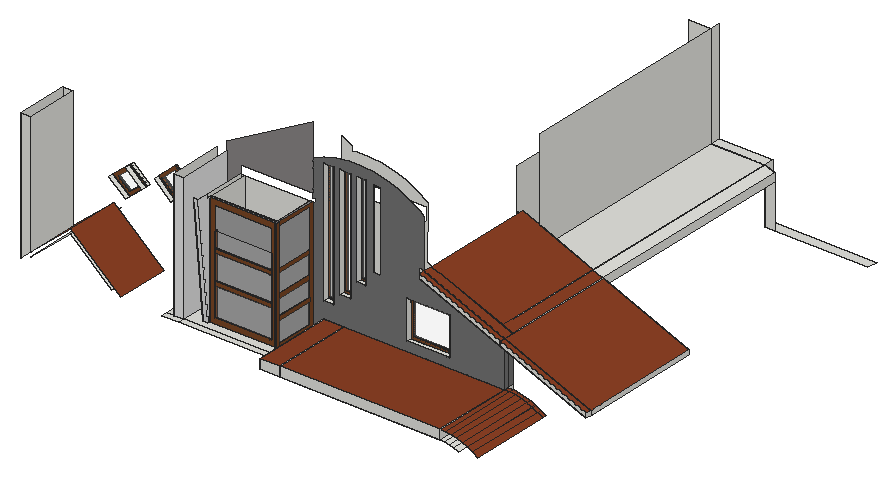
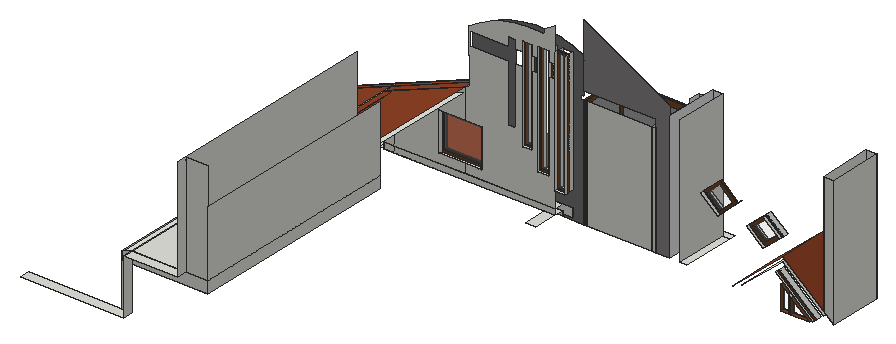
# SketchUp Ruby script. Lengths in inches.
U = 1.inch
M = Sketchup.active_model
def pt(a) = Geom::Point3d.new(a.map { |v| v * U })
def face(e, loops, mat)
  f = e.add_face(loops[0].map { |a| pt(a) })
  loops[1..].each { |l| e.add_face(l.map { |a| pt(a) }).erase! }
  f.material = f.back_material = mat if mat
  f
end
# faces: each face lists its corners as indices into pts; further lists are holes
def faces(e, pts, list, mat = nil) = list.each { |f| face(e, (f[0].is_a?(Array) ? f : [f]).map { |l| l.map { |i| pts[i] } }, mat) }
# xy, xz, yz: faces in a plane at the given z, y or x. An outline is a flat list of corners, or four numbers for a rectangle; further outlines are holes
def ring(l) = l.size == 4 ? [[l[0], l[1]], [l[2], l[1]], [l[2], l[3]], [l[0], l[3]]] : l.each_slice(2).to_a
def flat(e, list, mat, &to3) = list.each { |f| face(e, (f[0].is_a?(Array) ? f : [f]).map { |l| ring(l).map { |u, v| to3.(u, v) } }, mat) }
def xy(e, z, list, mat = nil) = flat(e, list, mat) { |x, y| [x, y, z] }
def xz(e, y, list, mat = nil) = flat(e, list, mat) { |x, z| [x, y, z] }
def yz(e, x, list, mat = nil) = flat(e, list, mat) { |y, z| [x, y, z] }
def lines(e, pts, list) = list.each { |a, b| e.add_line(pt(pts[a]), pt(pts[b])) }
# prism: a flat outline (further loops are holes) pulled along v
def prism(e, loops, v, mat = nil)
  f = face(e, loops, mat); d = Geom::Vector3d.new(v.map { |x| x * U })
  f.pushpull(f.normal.samedirection?(d) ? d.length : -d.length)
end
def box(e, o, s, mat = nil) = prism(e, [[o, [o[0] + s[0], o[1], o[2]], [o[0] + s[0], o[1] + s[1], o[2]], [o[0], o[1] + s[1], o[2]]]], [0, 0, s[2]], mat)
def at(x, y, z, deg = 0) = Geom::Transformation.translation(pt([x, y, z])) * Geom::Transformation.rotation(ORIGIN, Z_AXIS, deg.degrees)
def axes(o, x, y, z) = Geom::Transformation.new([*x, 0, *y, 0, *z, 0, *pt(o).to_a, 1])
def part(name) = M.definitions.add(name)
# library, detail: a bought-in or finely detailed component or shape, given as its bounding box
def library(name, o, s) = part(name).tap { |d| box(d.entities, o, s) }
def detail(e, o, s) = box(e.add_group.entities, o, s)
def put(e, d, t, mat = nil) = e.add_instance(d, t).tap { |i| i.material = mat if mat }
def group(e, t, mat = nil) = e.add_group.tap { |g| g.transformation = t; g.material = mat if mat }.entities
root = M.entities
M.materials.add("Glass Thin Clear 001").color = [243, 240, 240]
M.materials["Glass Thin Clear 001"].alpha = 0.1
M.materials.add("[Blinds Vertical Stripe Gray]").color = [160, 160, 160]
M.materials.add("[Brick Tumbled]").color = [135, 132, 132]
M.materials.add("[Color M01]").color = [226, 226, 226]
M.materials.add("[Color M05]").color = [114, 114, 114]
M.materials.add("[Roofing Tile Spanish]").color = [138, 64, 36]
M.materials.add("[Wood Veneer 01]").color = [120, 70, 37]
xy(root,124.49,[[41.61,170.5625,44.06,171.0625],[41.61,171.0625,44.06,173.875]])
xy(root,124.49,[[25.1,170.5625,41.61,171.0625],[44.06,170.5625,50.73,171.0625],[25.1,171.0625,41.61,173.875],[44.06,171.0625,50.73,173.875]],"[Wood Veneer 01]")
xy(root,126,[[141.15,112.5625,156.96,118.0625],[156.96,112.5625,252.96,118.0625],[141.15,118.0625,147.96,166.0625],[156.96,118.0625,252.96,118.0625,252.96,166.0625,233.59,166.0625,233.59,126.375,172.96,126.375,172.96,124.07,168.96,124.07,168.96,166.0625,156.96,166.0625],[252.96,118.0625,261.96,166.0625],
  [168.96,124.07,172.96,126.375],[168.96,126.375,172.96,166.0625],[172.96,126.375,231.27,128.3125],[231.84,126.375,233.59,128.3125],[172.96,128.3125,231.27,128.5625],
  [231.27,128.3125,231.84,128.5625],[231.84,128.3125,233.59,128.5625],[172.96,128.5625,231.27,128.9375],[172.96,128.9375,231.27,166.0625],[231.34,128.9375,231.84,166.0625]])
xy(root,126,[[231.27,126.375,231.84,128.3125],[231.27,128.5625,231.34,128.9375],[231.34,128.5625,231.84,128.9375],[231.84,128.5625,233.59,128.9375],[231.27,128.9375,231.34,166.0625],
  [231.84,128.9375,233.59,166.0625]],"[Wood Veneer 01]")
xy(root,127.6,[[244.09,93.6875,252.96,166.0625],[252.96,93.6875,261.96,118.0625],[261.96,93.6875,405.96,118.0625],[261.96,118.0625,405.96,166.0625]])
xy(root,128.55,[[231.27,128.93,233.15,163.51],[233.15,128.93,233.59,163.51]],"[Wood Veneer 01]")
xy(root,130.625,[[252.96,118.0625,261.96,166.0625],[261.96,118.0625,405.96,166.0625],[252.96,166.0625,261.96,175.0625],[261.96,166.0625,405.96,175.0625],[252.96,175.0625,261.96,196.0625],
  [396.96,469.0625,489.96,478.0625]])
xy(root,130.81,[[177.78,126.375,228.77,127],[177.78,127,228.77,128.9375]],"[Wood Veneer 01]")
xy(root,135.875,[[252.96,166.0625,333.96,175.0625],[333.96,166.0625,405.96,175.0625]])
xy(root,135.875,[[244.09,93.6875,261.96,166.0625],[261.96,93.6875,405.96,166.0625]],"[Roofing Tile Spanish]")
xy(root,144.3,[[318.48,166.0625,356.67,170.5625],[318.48,172.3125,356.67,175.0625]])
xy(root,144.3,[[318.48,170.5625,356.67,170.875],[318.48,170.875,356.67,171.8125],[318.48,171.8125,356.67,172.3125]],"[Wood Veneer 01]")
xy(root,146.54,[[320.73,170.5625,354.42,170.875],[320.73,170.875,354.42,172.3125]],"[Wood Veneer 01]")
xy(root,146.8,[[231.27,128.93,233.15,163.51],[233.15,128.93,233.59,163.51]],"[Wood Veneer 01]")
xy(root,150.38,[[231.27,128.93,233.15,163.51],[233.15,128.93,233.59,163.51]],"[Wood Veneer 01]")
xy(root,150.4,[[243.5625,166.0625,252.8125,170.5625],[243.5625,172.5,252.8125,175.0625]])
xy(root,150.4,[[243.5625,170.5625,252.8125,172.125],[243.5625,172.125,252.8125,172.5]],"[Wood Veneer 01]")
xy(root,151.26,[[244.43,170.5625,251.95,170.8125],[244.43,170.8125,251.95,172.5]],"[Wood Veneer 01]")
xy(root,156.93,[[177.78,126.375,228.77,127],[177.78,127,228.77,128.9375]],"[Wood Veneer 01]")
xy(root,160.3125,[[177.78,126.375,228.77,127],[177.78,127,228.77,128.9375]],"[Wood Veneer 01]")
xy(root,160.43,[[258.23,166.0625,268.1,170.5625],[258.23,170.5625,268.1,172.4375],[258.23,172.4375,268.1,172.5],[258.23,172.5,268.1,175.0625]])
xy(root,161.64,[[259.4375,170.5625,266.9,171.125],[259.4375,171.125,266.9,172.5]],"[Wood Veneer 01]")
xy(root,164.87,[[231.27,128.93,233.15,163.51],[233.15,128.93,233.59,163.51]],"[Wood Veneer 01]")
xy(root,168.44,[[231.27,128.93,233.15,163.51],[233.15,128.93,233.59,163.51]],"[Wood Veneer 01]")
xy(root,170.02,[[328.85,276.6875,396.96,469.0625],[396.96,276.6875,405.96,469.0625]])
xy(root,175.79,[[273.05,166.0625,281.55,170.5625],[273.05,170.5625,281.55,172.4375],[273.05,172.4375,281.55,172.5],[273.05,172.5,281.55,175.0625]])
xy(root,176.74,[[320.73,170.5625,354.42,170.875],[320.73,170.875,354.42,172.3125]],"[Wood Veneer 01]")
xy(root,176.78,[[274.03,170.5625,280.57,171.125],[274.03,171.125,280.57,172.5]],"[Wood Veneer 01]")
xy(root,177,[[396.96,175.0625,405.96,187.0625],[396.96,187.0625,405.96,276.6875]])
xy(root,178.98,[[318.48,166.0625,356.67,170.5625],[318.48,172.3125,356.67,175.0625]])
xy(root,178.98,[[318.48,170.5625,356.67,170.875],[318.48,170.875,356.67,171.8125],[318.48,171.8125,356.67,172.3125]],"[Wood Veneer 01]")
xy(root,180.58,[[328.85,276.6875,348.92,469.0625],[348.92,276.6875,396.96,469.0625],[348.92,469.0625,396.96,478.0625]])
xy(root,183.04,[[177.78,126.375,228.77,127],[177.78,127,228.77,128.9375]],"[Wood Veneer 01]")
xy(root,185.43,[[231.27,128.93,233.15,163.51],[233.15,128.93,233.59,163.51]],"[Wood Veneer 01]")
xy(root,186.43,[[177.78,126.375,228.77,127],[177.78,127,228.77,128.9375]],"[Wood Veneer 01]")
xz(root,93.6875,[[244.09,127.6,261.96,135.875],[261.96,127.6,405.96,135.875]])
xz(root,118.0625,[[9.96,124,18.96,131.72,18.96,240,9.96,240],[252.96,126,261.96,127.6],[252.96,127.6,261.96,130.625],[261.96,127.6,405.96,130.625]])
xz(root,118.0625,[[147.96,126,156.96,240]],"[Color M01]")
xz(root,126.375,[[168.96,126,172.96,226.125]])
xz(root,126.375,[[[172.96,126,231.27,226.125],[177.78,130.81,228.77,221.31]],[231.27,126,231.84,226.125],[231.84,126,233.59,226.125],[177.78,156.93,228.77,160.3125],[177.78,183.04,228.77,186.43]],"[Wood Veneer 01]")
xz(root,127,[[177.78,130.81,228.77,156.93],[177.78,160.3125,228.77,183.04],[177.78,186.43,228.77,200.48]],"Glass Thin Clear 001")
xz(root,128.3125,[[172.96,126,233.59,226.125]],"[Blinds Vertical Stripe Gray]")
xz(root,128.93,[[231.27,146.8,233.59,150.38],[231.27,164.87,233.59,168.44],[231.27,185.43,233.59,189.01]])
xz(root,128.93,[[231.27,128.55,233.15,146.8],[233.15,128.55,233.59,146.8],[231.27,150.38,233.15,164.87],[233.15,150.38,233.59,164.87],[231.27,168.44,233.15,185.43],
  [233.15,168.44,233.59,185.43]],"[Wood Veneer 01]")
xz(root,128.9375,[[[172.96,126,233.59,226.125],[177.78,130.81,228.77,221.31]],[177.78,156.93,228.77,160.3125],[177.78,183.04,228.77,186.43]],"[Wood Veneer 01]")
xz(root,161.1875,[[483.0625,142.27,483.0625,146.27,405.96,177,405.96,173],[405.96,173,405.96,177,333.96,205.6875,333.96,201.6875]])
xz(root,163.51,[[231.27,146.8,233.59,150.38],[231.27,164.87,233.59,168.44],[231.27,185.43,233.59,189.01]])
xz(root,163.51,[[231.27,128.55,233.15,146.8],[233.15,128.55,233.59,146.8],[231.27,150.38,233.15,164.87],[233.15,150.38,233.59,164.87],[231.27,168.44,233.15,185.43],
  [233.15,168.44,233.59,185.43]],"[Wood Veneer 01]")
xz(root,166.0625,[[9.96,124,9.96,240,18.96,240,18.96,131.72],[168.96,126,172.96,226.125],[172.96,126,231.27,226.125],[231.34,126,231.84,226.125],[252.96,126,261.96,130.625],
  [244.09,127.6,244.09,135.875,261.96,135.875,261.96,130.625,252.96,130.625,252.96,127.6],[261.96,127.6,405.96,130.625],[261.96,130.625,405.96,135.875],[483.0625,142.27,405.96,173,405.96,177,483.0625,146.27],[405.96,173,333.96,201.6875,333.96,205.6875,405.96,177]])
xz(root,166.0625,[[156.96,126,168.96,126,168.96,233.5,233.59,233.5,233.59,290.5,156.96,248]],"[Brick Tumbled]")
xz(root,166.0625,[[[233.59,126,252.96,126,252.96,127.6,244.09,127.6,244.09,135.875,405.96,135.875,405.96,173,333.96,201.6875,328.85,203.72,328.85,207.72,333.96,205.6875,333.96,249.1,329.8,252.53,320.33,258.625,310.2,263.55,299.57,267.25,288.57,269.67,277.36,270.78,266.11,270.55,261.96,269.97,254.95,268.99,252.96,268.47,244.0625,266.13,233.59,262,233.59,229.5625,236.34,229.5625,236.34,226.125,233.59,226.125],[318.48,144.3,356.67,178.98],[243.5625,150.4,252.8125,261.4],[258.23,160.43,268.1,261.18],[273.05,175.79,281.55,260.67],[288.03,188.71,295.34,259.58]]],"[Color M05]")
xz(root,166.0625,[[231.27,126,231.34,226.125],[231.84,126,233.59,226.125]],"[Wood Veneer 01]")
xz(root,170.5625,[[41.61,124.49,44.06,124.49,44.06,140.36,41.61,138.3],[[318.48,144.3,356.67,178.98],[320.73,146.54,354.42,176.74]],[[243.5625,150.4,252.8125,261.4],[244.43,151.26,251.95,260.53]],[[258.23,160.43,268.1,261.18],[259.4375,161.64,266.9,259.97]],[[66.04,170.09,80.79,182.43,66.04,194.78,51.29,182.43],[66.04,173.375,55.21,182.43,66.04,191.49,76.86,182.43]],
  [[273.05,175.79,281.55,260.67],[274.03,176.78,280.57,259.6875]],[[106.65,181.57,121.43,195.01,106.65,208.45,91.87,195.01],[106.65,184.29,94.86,195.01,106.65,205.73,118.44,195.01]]],"[Wood Veneer 01]")
xz(root,170.8125,[[244.43,151.26,251.95,260.53]],"Glass Thin Clear 001")
xz(root,170.875,[[[318.48,144.3,356.67,178.98],[320.73,146.54,354.42,176.74]]])
xz(root,170.875,[[320.73,146.54,354.42,176.74],[66.04,173.375,76.86,182.43,66.04,191.49,55.21,182.43],[106.65,184.29,118.44,195.01,106.65,205.73,94.86,195.01]],"Glass Thin Clear 001")
xz(root,171.0625,[[41.61,124.49,41.61,138.3,44.06,140.36,44.06,124.49]])
xz(root,171.0625,[[25.1,124.49,41.61,124.49,41.61,138.3],[44.06,124.49,50.73,124.49,50.73,145.9375,44.06,140.36]],"Glass Thin Clear 001")
xz(root,171.125,[[259.4375,161.64,266.9,259.97],[274.03,176.78,280.57,259.6875]],"Glass Thin Clear 001")
xz(root,171.8125,[[318.48,144.3,356.67,178.98]],"Glass Thin Clear 001")
xz(root,171.875,[[66.04,170.09,51.29,182.43,66.04,194.78,80.79,182.43],[106.65,181.57,91.87,195.01,106.65,208.45,121.43,195.01]],"Glass Thin Clear 001")
xz(root,172.125,[[243.5625,150.4,252.8125,261.4]],"Glass Thin Clear 001")
xz(root,172.3125,[[[318.48,144.3,356.67,178.98],[320.73,146.54,354.42,176.74]]],"[Wood Veneer 01]")
xz(root,172.4375,[[258.23,160.43,268.1,261.18],[273.05,175.79,281.55,260.67]],"Glass Thin Clear 001")
xz(root,172.4375,[[[66.04,170.09,51.29,182.43,66.04,194.78,80.79,182.43],[66.04,173.375,76.86,182.43,66.04,191.49,55.21,182.43]],[[106.65,181.57,91.87,195.01,106.65,208.45,121.43,195.01],[106.65,184.29,118.44,195.01,106.65,205.73,94.86,195.01]]],"[Wood Veneer 01]")
xz(root,172.5,[[[243.5625,150.4,252.8125,261.4],[244.43,151.26,251.95,260.53]],[[258.23,160.43,268.1,261.18],[259.4375,161.64,266.9,259.97]],[[273.05,175.79,281.55,260.67],[274.03,176.78,280.57,259.6875]]],"[Wood Veneer 01]")
xz(root,173.875,[[41.61,124.49,41.61,138.3,44.06,140.36,44.06,124.49]],"[Wood Veneer 01]")
xz(root,175.0625,[[252.96,130.625,396.96,135.875],[396.96,130.625,405.96,135.875],[252.96,135.875,252.96,240,258.23,240,258.23,160.43,268.1,160.43,268.1,240,273.05,240,273.05,175.79,281.55,175.79,281.55,240,288.03,240,288.03,188.71,295.34,188.71,295.34,240,328.85,240,328.85,252,295.34,252,295.34,259.58,288.03,259.58,288.03,252,281.55,252,281.55,260.67,273.05,260.67,273.05,252,268.1,252,268.1,261.18,258.23,261.18,258.23,252,252.96,252,252.96,282.53,261.96,276.98,261.96,272.98,266.11,273.55,277.36,273.78,288.57,272.68,299.57,270.26,310.2,266.5625,320.33,261.63,329.8,255.54,328.85,207.72,333.96,205.6875,333.96,178.98,318.48,178.98,318.48,144.3,333.96,144.3,333.96,135.875],[333.96,135.875,333.96,144.3,356.67,144.3,356.67,178.98,333.96,178.98,333.96,205.6875,396.96,180.58,396.96,135.875],[396.96,135.875,405.96,177],
  [396.96,177,405.96,177,396.96,180.58]])
xz(root,276.6875,[[483.0625,142.27,405.96,173,405.96,177,483.0625,146.27],[328.85,170.02,396.96,176.58],[396.96,170.02,405.96,170.02,405.96,173,396.96,176.58],[405.96,173,396.96,176.58,396.96,177,405.96,177],[328.85,176.58,396.96,176.58,395.92,177,328.85,177],
  [396.96,176.58,395.92,177,396.96,177],[328.85,177,395.92,177,386.92,180.58,328.85,180.58],[395.92,177,386.92,180.58,396.96,180.58,396.96,177],[396.96,177,405.96,177,396.96,180.58],[328.85,180.58,348.92,180.58,348.92,195.73,333.96,201.6875,328.85,203.72],
  [386.92,180.58,348.92,195.73,348.92,199.73,396.96,180.58]])
xz(root,469.0625,[[396.96,130.625,405.96,170.02],[328.85,170.02,396.96,180.58],[396.96,170.02,396.96,180.58,405.96,177,405.96,170.02],[328.85,180.58,348.92,272.68]])
yz(root,9.96,[[118.0625,124,166.0625,240]])
yz(root,18.96,[[118.0625,131.72,166.0625,240]])
yz(root,41.61,[[170.5625,124.49,171.0625,138.3],[171.0625,124.49,173.875,138.3]],"[Wood Veneer 01]")
yz(root,44.06,[[170.5625,124.49,171.0625,140.36],[171.0625,124.49,173.875,140.36]],"[Wood Veneer 01]")
yz(root,50.73,[[170.5625,124.49,171.0625,145.9375],[171.0625,124.49,173.875,145.9375]],"[Wood Veneer 01]")
yz(root,147.96,[[118.0625,126,166.0625,240]])
yz(root,156.96,[[118.0625,126,166.0625,240]],"[Color M01]")
yz(root,168.96,[[124.07,126,113.91,226.125,126.375,226.125,126.375,126],[126.375,126,166.0625,226.125]])
yz(root,172.96,[[128.3125,126,128.5625,226.125],[128.9375,126,166.0625,226.125]])
yz(root,172.96,[[124.07,126,126.375,126,126.375,226.125,123.625,226.125,123.625,229.5625,113.5625,229.5625]],"[Color M01]")
yz(root,172.96,[[126.375,126,128.3125,226.125],[128.5625,126,128.9375,226.125]],"[Wood Veneer 01]")
yz(root,177.78,[[126.375,156.93,128.9375,160.3125],[126.375,183.04,128.9375,186.43]])
yz(root,177.78,[[126.375,130.81,127,156.93],[127,130.81,128.9375,156.93],[126.375,160.3125,127,183.04],[127,160.3125,128.9375,183.04],[126.375,186.43,127,200.48],
  [127,186.43,128.9375,200.48]],"[Wood Veneer 01]")
yz(root,228.77,[[126.375,156.93,128.9375,160.3125],[126.375,183.04,128.9375,186.43]])
yz(root,228.77,[[126.375,130.81,127,156.93],[127,130.81,128.9375,156.93],[126.375,160.3125,127,183.04],[127,160.3125,128.9375,183.04],[126.375,186.43,127,200.48],
  [127,186.43,128.9375,200.48]],"[Wood Veneer 01]")
yz(root,231.27,[[[126.375,126,166.0625,226.125],[128.93,128.55,163.51,223.57]],[128.93,146.8,163.51,150.38],[128.93,164.87,163.51,168.44],[128.93,185.43,163.51,189.01]],"[Wood Veneer 01]")
yz(root,231.84,[[126.375,126,166.0625,226.125]],"[Blinds Vertical Stripe Gray]")
yz(root,233.15,[[128.93,128.55,163.51,146.8],[128.93,150.38,163.51,164.87],[128.93,168.44,163.51,185.43]],"Glass Thin Clear 001")
yz(root,233.59,[[126.375,126,128.3125,226.125],[128.3125,126,128.9375,126,128.9375,128.55,128.93,128.55,128.93,223.57,128.9375,223.57,128.9375,226.125,128.3125,226.125],[128.9375,126,166.0625,126,166.0625,226.125,128.9375,226.125,128.9375,223.57,163.51,223.57,163.51,128.55,128.9375,128.55],[128.93,128.55,128.9375,146.8],[128.93,146.8,128.9375,150.38],
  [128.9375,146.8,163.51,150.38],[128.93,150.38,128.9375,164.87],[128.93,164.87,128.9375,168.44],[128.9375,164.87,163.51,168.44],[128.93,168.44,128.9375,185.43],
  [128.93,185.43,128.9375,189.01],[128.9375,185.43,163.51,189.01]],"[Wood Veneer 01]")
yz(root,243.5625,[[166.0625,150.4,170.5625,261.4],[172.5,150.4,175.0625,261.4]])
yz(root,243.5625,[[170.5625,150.4,172.125,261.4],[172.125,150.4,172.5,261.4]],"[Wood Veneer 01]")
yz(root,244.09,[[93.6875,127.6,166.0625,135.875]])
yz(root,244.43,[[170.5625,151.26,170.8125,260.53],[170.8125,151.26,172.5,260.53]],"[Wood Veneer 01]")
yz(root,251.95,[[170.5625,151.26,170.8125,260.53],[170.8125,151.26,172.5,260.53]],"[Wood Veneer 01]")
yz(root,252.8125,[[166.0625,150.4,170.5625,261.4],[172.5,150.4,175.0625,261.4]])
yz(root,252.8125,[[170.5625,150.4,172.125,261.4],[172.125,150.4,172.5,261.4]],"[Wood Veneer 01]")
yz(root,252.96,[[118.0625,126,166.0625,127.6],[118.0625,127.6,166.0625,130.625]])
yz(root,258.23,[[166.0625,160.43,170.5625,261.18],[172.5,160.43,175.0625,261.18]])
yz(root,258.23,[[170.5625,160.43,172.4375,261.18],[172.4375,160.43,172.5,261.18]],"[Wood Veneer 01]")
yz(root,259.4375,[[170.5625,161.64,171.125,259.97],[171.125,161.64,172.5,259.97]],"[Wood Veneer 01]")
yz(root,261.96,[[118.0625,126,166.0625,127.6],[93.6875,127.6,93.6875,135.875,166.0625,135.875,166.0625,130.625,118.0625,130.625,118.0625,127.6],[118.0625,127.6,166.0625,130.625]])
yz(root,266.9,[[170.5625,161.64,171.125,259.97],[171.125,161.64,172.5,259.97]],"[Wood Veneer 01]")
yz(root,268.1,[[166.0625,160.43,170.5625,261.18],[172.5,160.43,175.0625,261.18]])
yz(root,268.1,[[170.5625,160.43,172.4375,261.18],[172.4375,160.43,172.5,261.18]],"[Wood Veneer 01]")
yz(root,273.05,[[166.0625,175.79,170.5625,260.67],[172.5,175.79,175.0625,260.67]])
yz(root,273.05,[[170.5625,175.79,172.4375,260.67],[172.4375,175.79,172.5,260.67]],"[Wood Veneer 01]")
yz(root,274.03,[[170.5625,176.78,171.125,259.6875],[171.125,176.78,172.5,259.6875]],"[Wood Veneer 01]")
yz(root,280.57,[[170.5625,176.78,171.125,259.6875],[171.125,176.78,172.5,259.6875]],"[Wood Veneer 01]")
yz(root,281.55,[[166.0625,175.79,170.5625,260.67],[172.4375,175.79,172.5,260.67],[172.5,175.79,175.0625,260.67]])
yz(root,281.55,[[170.5625,175.79,172.4375,260.67]],"[Wood Veneer 01]")
yz(root,318.48,[[166.0625,144.3,170.5625,178.98],[172.3125,144.3,175.0625,178.98]])
yz(root,318.48,[[170.5625,144.3,170.875,178.98],[170.875,144.3,171.8125,178.98],[171.8125,144.3,172.3125,178.98]],"[Wood Veneer 01]")
yz(root,320.73,[[170.5625,146.54,170.875,176.74],[170.875,146.54,172.3125,176.74]],"[Wood Veneer 01]")
yz(root,328.85,[[276.6875,170.02,469.0625,180.58],[276.6875,180.58,469.0625,240]])
yz(root,348.92,[[276.6875,180.58,469.0625,272.68],[469.0625,180.58,478.0625,272.68]])
yz(root,354.42,[[170.5625,146.54,170.875,176.74],[170.875,146.54,172.3125,176.74]],"[Wood Veneer 01]")
yz(root,356.67,[[166.0625,144.3,170.5625,178.98],[172.3125,144.3,175.0625,178.98]])
yz(root,356.67,[[170.5625,144.3,170.875,178.98],[170.875,144.3,171.8125,178.98],[171.8125,144.3,172.3125,178.98]],"[Wood Veneer 01]")
yz(root,396.96,[[469.0625,130.625,478.0625,180.58],[276.6875,170.02,469.0625,180.58],[187.0625,177,196.0625,180.58],[196.0625,177,276.6875,180.58]])
yz(root,405.96,[[93.6875,127.6,93.6875,135.875,166.0625,135.875,166.0625,130.625,118.0625,130.625,118.0625,127.6],[118.0625,127.6,166.0625,130.625],[166.0625,127.6,169.5,130.625],[166.0625,130.625,169.5,135.875],[169.5,130.625,175.0625,135.875],
  [276.6875,170.02,469.0625,177],[161.1875,173,166.0625,177],[166.0625,173,169.5,177],[169.5,173,175.0625,177],[175.0625,173,187.0625,177],
  [187.0625,173,276.6875,177]])
yz(root,405.96,[[166.0625,135.875,169.5,173],[169.5,135.875,175.0625,173]],"[Color M05]")
yz(root,483.0625,[[161.1875,142.27,166.0625,146.27],[166.0625,142.27,276.6875,146.27]])
p = [[418.82,93.6875,125.42],[418.82,166.0625,125.42],[422.91,166.0625,123.88],[422.91,93.6875,123.88],[418.82,169.5,125.42],[422.91,169.5,123.88],
  [18.96,166.0625,131.72],[9.96,166.0625,124],[9.96,118.0625,124],[18.96,118.0625,131.72],[99.96,166.0625,124],[55.42,166.0625,163],
  [55.42,118.0625,163],[99.96,118.0625,124],[25.1,171.0625,124.49],[41.61,171.0625,138.3],[41.61,170.5625,138.3],[25.1,170.5625,124.49],
  [41.61,173.875,138.3],[25.1,173.875,124.49],[440.24,93.6875,125.125],[440.24,166.0625,125.125],[435.87,166.0625,127.97],[435.87,93.6875,127.97],
  [440.24,169.5,125.125],[435.87,169.5,127.97],[414.61,93.6875,126.55],[414.61,166.0625,126.55],[414.61,169.5,126.55],[172.96,124.07,126],
  [172.96,113.5625,229.5625],[168.96,113.5625,229.5625],[168.96,113.91,226.125],[168.96,124.07,126],[21.04,166.0625,126.39],[21.04,170.5625,126.39],
  [54.79,170.5625,154.64],[54.79,166.0625,154.64],[54.79,171.0625,154.64],[21.04,171.0625,126.39],[54.79,173.0625,154.64],[21.04,173.0625,126.39],
  [21.04,173.875,126.39],[54.79,173.875,154.64],[54.79,175.0625,154.64],[21.04,175.0625,126.39],[410.3125,93.6875,127.28],[410.3125,166.0625,127.28],
  [410.3125,169.5,127.28],[55.42,166.0625,159],[91.87,166.0625,127.08],[91.87,118.0625,127.08],[55.42,118.0625,159],[405.96,118.0625,127.6],
  [405.96,166.0625,127.6],[405.96,93.6875,127.6],[405.96,169.5,127.6],[18.96,166.0625,127.72],[18.96,118.0625,127.72],[431.26,166.0625,130.42],
  [431.26,93.6875,130.42],[431.26,169.5,130.42],[430.75,166.0625,130.625],[430.75,93.6875,130.625],[430.75,169.5,130.625],[426.4375,166.0625,132.43],
  [426.4375,93.6875,132.43],[426.4375,169.5,132.43],[421.46,166.0625,133.99],[421.46,93.6875,133.99],[421.46,169.5,133.99],[416.36,166.0625,135.09],
  [416.36,93.6875,135.09],[416.36,169.5,135.09],[411.18,166.0625,135.72],[411.18,93.6875,135.72],[411.18,169.5,135.72],[405.96,166.0625,135.875],
  [405.96,93.6875,135.875],[405.96,169.5,135.875],[44.06,170.5625,140.36],[44.06,171.0625,140.36],[44.06,173.875,140.36],[50.73,171.0625,145.9375],
  [50.73,170.5625,145.9375],[50.73,173.875,145.9375],[405.96,166.0625,173],[483.0625,166.0625,142.27],[483.0625,161.1875,142.27],[405.96,161.1875,173],
  [483.0625,276.6875,142.27],[405.96,169.5,173],[405.96,175.0625,173],[405.96,187.0625,173],[405.96,276.6875,173],[483.0625,166.0625,146.27],
  [405.96,166.0625,177],[405.96,161.1875,177],[483.0625,161.1875,146.27],[405.96,169.5,177],[483.0625,276.6875,146.27],[405.96,276.6875,177],
  [405.96,187.0625,177],[405.96,175.0625,177],[66.04,166.0625,170.09],[66.04,170.5625,170.09],[51.29,170.5625,182.43],[51.29,166.0625,182.43],
  [80.79,166.0625,182.43],[80.79,170.5625,182.43],[51.29,171.875,182.43],[66.04,171.875,170.09],[80.79,171.875,182.43],[66.04,172.4375,170.09],
  [51.29,172.4375,182.43],[80.79,172.4375,182.43],[51.29,175.0625,182.43],[66.04,175.0625,170.09],[80.79,175.0625,182.43],[333.96,166.0625,201.6875],
  [333.96,161.1875,201.6875],[333.96,175.0625,201.6875],[333.96,276.6875,201.6875],[348.92,276.6875,195.73],[386.92,276.6875,180.58],[395.92,276.6875,177],
  [396.96,276.6875,176.58],[66.04,170.875,173.375],[55.21,170.875,182.43],[55.21,170.5625,182.43],[66.04,170.5625,173.375],[76.86,170.875,182.43],
  [76.86,170.5625,182.43],[55.21,172.4375,182.43],[66.04,172.4375,173.375],[76.86,172.4375,182.43],[333.96,166.0625,205.6875],[333.96,161.1875,205.6875],
  [396.96,175.0625,180.58],[333.96,175.0625,205.6875],[396.96,187.0625,180.58],[396.96,276.6875,180.58],[396.96,196.0625,180.58],[405.96,469.0625,177],
  [396.96,469.0625,180.58],[333.96,276.6875,205.6875],[348.92,276.6875,199.73],[106.65,166.0625,181.57],[106.65,170.5625,181.57],[91.87,170.5625,195.01],
  [91.87,166.0625,195.01],[121.43,166.0625,195.01],[121.43,170.5625,195.01],[91.87,171.875,195.01],[106.65,171.875,181.57],[121.43,171.875,195.01],
  [106.65,172.4375,181.57],[91.87,172.4375,195.01],[121.43,172.4375,195.01],[91.87,175.0625,195.01],[106.65,175.0625,181.57],[121.43,175.0625,195.01],
  [66.04,170.5625,194.78],[66.04,166.0625,194.78],[66.04,171.875,194.78],[66.04,170.875,191.49],[66.04,170.5625,191.49],[66.04,172.4375,191.49],
  [66.04,172.4375,194.78],[66.04,175.0625,194.78],[106.65,170.875,184.29],[94.86,170.875,195.01],[94.86,170.5625,195.01],[106.65,170.5625,184.29],
  [118.44,170.875,195.01],[118.44,170.5625,195.01],[94.86,172.4375,195.01],[106.65,172.4375,184.29],[118.44,172.4375,195.01]]
faces(root,p,[[0,1,2,3],[2,1,4,5],[6,7,8,9],[26,27,1,0],[1,27,28,4],[34,35,36,37],[44,43,42,45],[46,47,27,26],
  [27,47,48,28],[49,50,51,52],[53,54,47,46,55],[47,54,56,48],[57,49,52,58],[16,80,81,15],[81,82,18,15],[86,87,88,89],
  [90,87,86,91,92,93,94],[104,105,106,107],[108,109,105,104],[116,114,113,117],[117,113,115,118],[119,86,89,120],[91,86,119,121,122,123,124,125,126,94,93,92],[141,101,143,144],
  [147,148,149,150],[151,152,148,147],[159,157,156,160],[160,156,158,161],[107,106,162,163],[163,162,109,108],[169,168,114,116],[118,115,168,169],
  [170,171,172,173]])
faces(root,p,[[10,11,12,13],[20,21,22,23],[22,21,24,25],[23,22,59,60],[59,22,25,61],[60,59,62,63],[62,59,61,64],[63,62,65,66],
  [65,62,64,67],[11,6,9,12],[66,65,68,69],[68,65,67,70],[69,68,71,72],[71,68,70,73],[72,71,74,75],[74,71,73,76],
  [75,74,77,78],[77,74,76,79],[95,96,97,98],[99,96,95,100,101,102,103],[96,136,137,97],[136,96,99,103,138,139],[140,138,103,102,101,141,142],[145,139,138,140,142,141,146]],"[Roofing Tile Spanish]")
faces(root,p,[[14,15,16,17],[18,15,14,19],[38,39,35,36],[40,41,39,38],[42,41,40,43],[81,83,84,80],[85,83,81,82],[110,111,105,106],
  [111,112,109,105],[113,111,110,114],[115,112,111,113],[127,128,129,130],[131,127,130,132],[133,128,127,134],[134,127,131,135],[153,154,148,149],
  [154,155,152,148],[156,154,153,157],[158,155,154,156],[164,110,106,162],[128,165,166,129],[112,164,162,109],[165,131,132,166],[167,165,128,133],
  [135,131,165,167],[114,110,164,168],[168,164,112,115],[174,170,173,175],[176,171,170,177],[177,170,174,178]],"[Wood Veneer 01]")
faces(root,p,[[29,30,31,32,33]],"[Color M01]")
